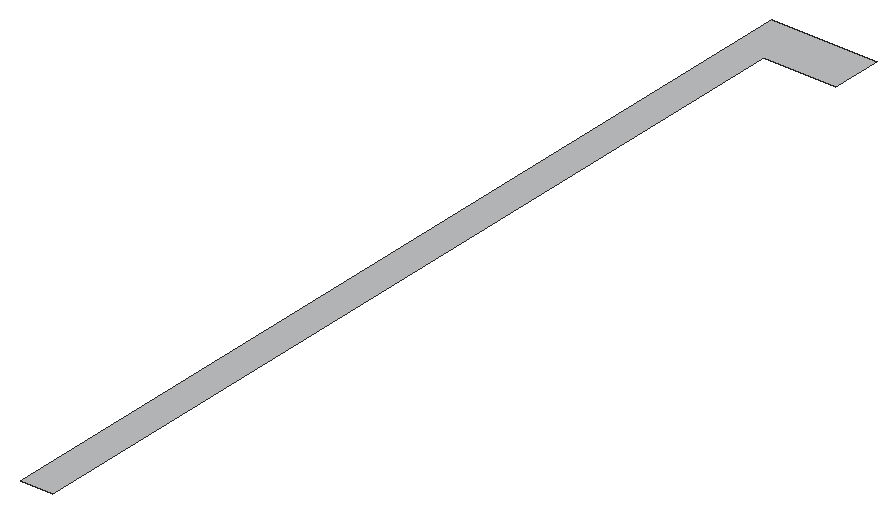
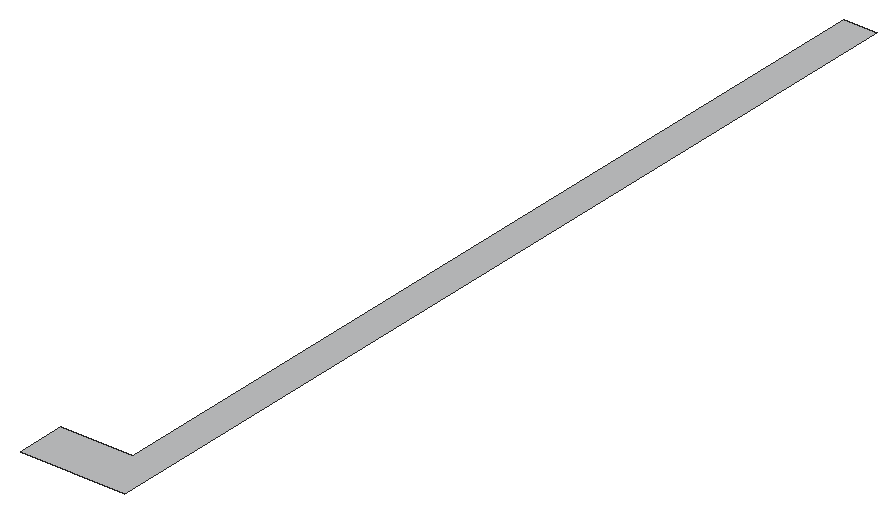
# SketchUp Ruby script. Lengths in inches.
U = 1.inch
M = Sketchup.active_model
def pt(a) = Geom::Point3d.new(a.map { |v| v * U })
def face(e, loops, mat)
  f = e.add_face(loops[0].map { |a| pt(a) })
  loops[1..].each { |l| e.add_face(l.map { |a| pt(a) }).erase! }
  f.material = f.back_material = mat if mat
  f
end
# faces: each face lists its corners as indices into pts; further lists are holes
def faces(e, pts, list, mat = nil) = list.each { |f| face(e, (f[0].is_a?(Array) ? f : [f]).map { |l| l.map { |i| pts[i] } }, mat) }
# xy, xz, yz: faces in a plane at the given z, y or x. An outline is a flat list of corners, or four numbers for a rectangle; further outlines are holes
def ring(l) = l.size == 4 ? [[l[0], l[1]], [l[2], l[1]], [l[2], l[3]], [l[0], l[3]]] : l.each_slice(2).to_a
def flat(e, list, mat, &to3) = list.each { |f| face(e, (f[0].is_a?(Array) ? f : [f]).map { |l| ring(l).map { |u, v| to3.(u, v) } }, mat) }
def xy(e, z, list, mat = nil) = flat(e, list, mat) { |x, y| [x, y, z] }
def xz(e, y, list, mat = nil) = flat(e, list, mat) { |x, z| [x, y, z] }
def yz(e, x, list, mat = nil) = flat(e, list, mat) { |y, z| [x, y, z] }
def lines(e, pts, list) = list.each { |a, b| e.add_line(pt(pts[a]), pt(pts[b])) }
# prism: a flat outline (further loops are holes) pulled along v
def prism(e, loops, v, mat = nil)
  f = face(e, loops, mat); d = Geom::Vector3d.new(v.map { |x| x * U })
  f.pushpull(f.normal.samedirection?(d) ? d.length : -d.length)
end
def box(e, o, s, mat = nil) = prism(e, [[o, [o[0] + s[0], o[1], o[2]], [o[0] + s[0], o[1] + s[1], o[2]], [o[0], o[1] + s[1], o[2]]]], [0, 0, s[2]], mat)
def at(x, y, z, deg = 0) = Geom::Transformation.translation(pt([x, y, z])) * Geom::Transformation.rotation(ORIGIN, Z_AXIS, deg.degrees)
def axes(o, x, y, z) = Geom::Transformation.new([*x, 0, *y, 0, *z, 0, *pt(o).to_a, 1])
def part(name) = M.definitions.add(name)
# library, detail: a bought-in or finely detailed component or shape, given as its bounding box
def library(name, o, s) = part(name).tap { |d| box(d.entities, o, s) }
def detail(e, o, s) = box(e.add_group.entities, o, s)
def put(e, d, t, mat = nil) = e.add_instance(d, t).tap { |i| i.material = mat if mat }
def group(e, t, mat = nil) = e.add_group.tap { |g| g.transformation = t; g.material = mat if mat }.entities
root = M.entities
M.materials.add("[Fencing Metal Straight]").color = [194, 195, 196]
xy(root,115.1875,[[0,0,14.48,0,14.48,390.99,46.1875,390.99,46.1875,413.49,0,413.49]],"[Fencing Metal Straight]")
